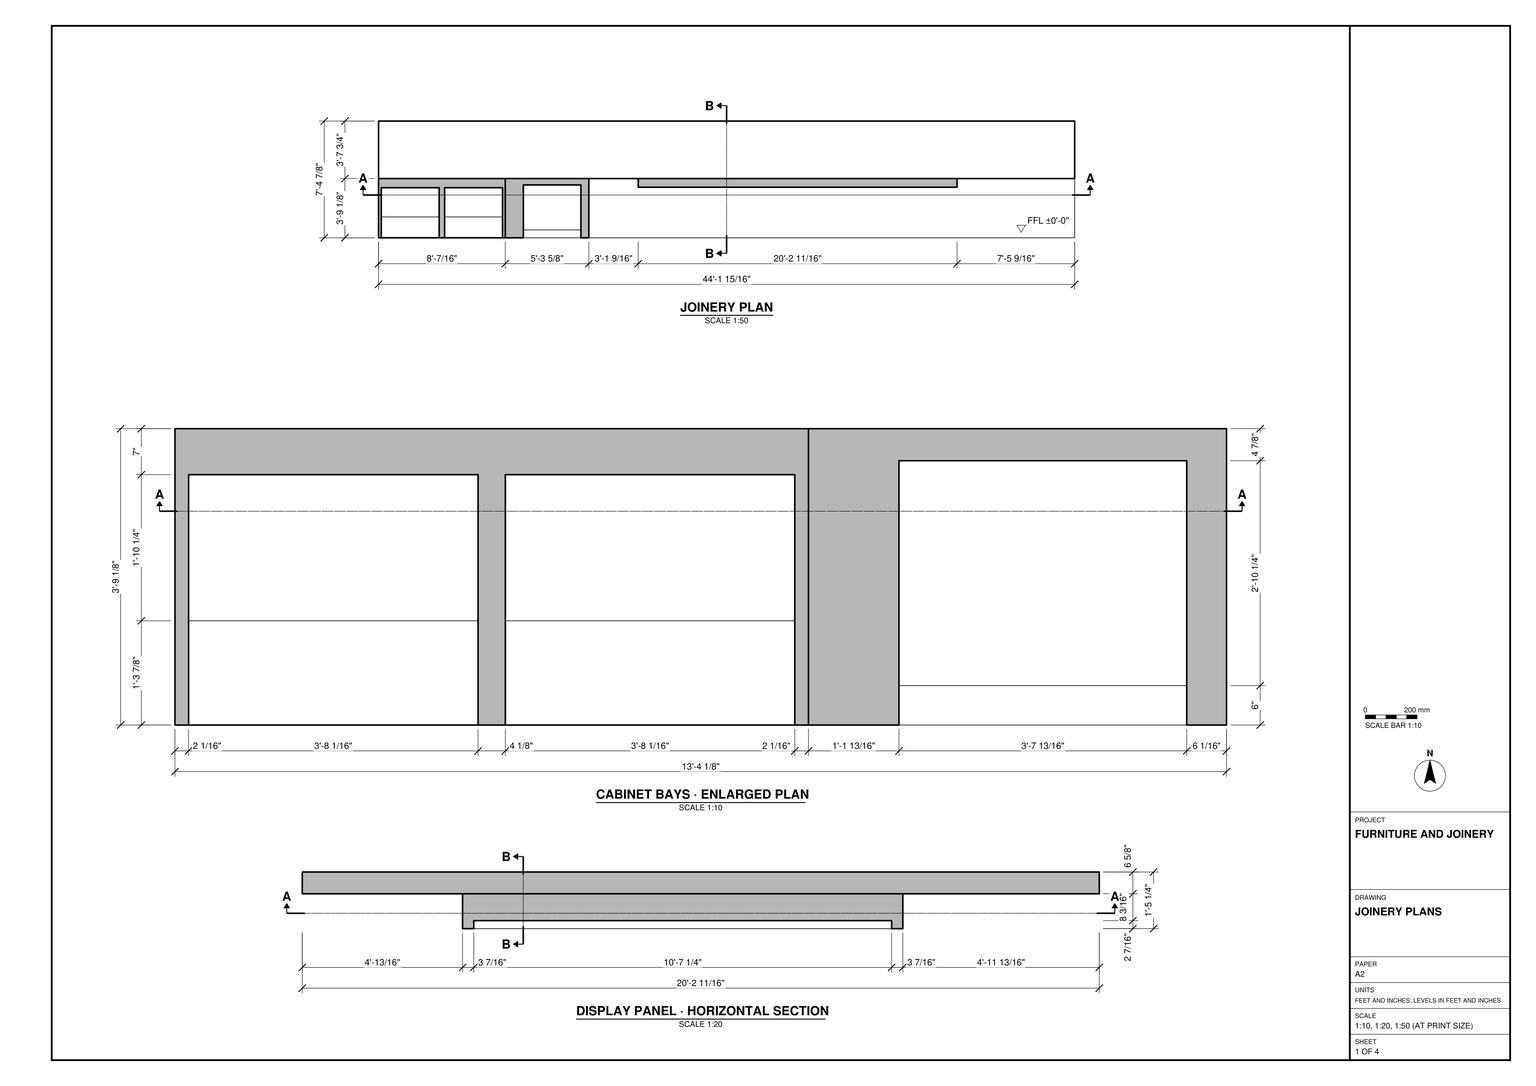
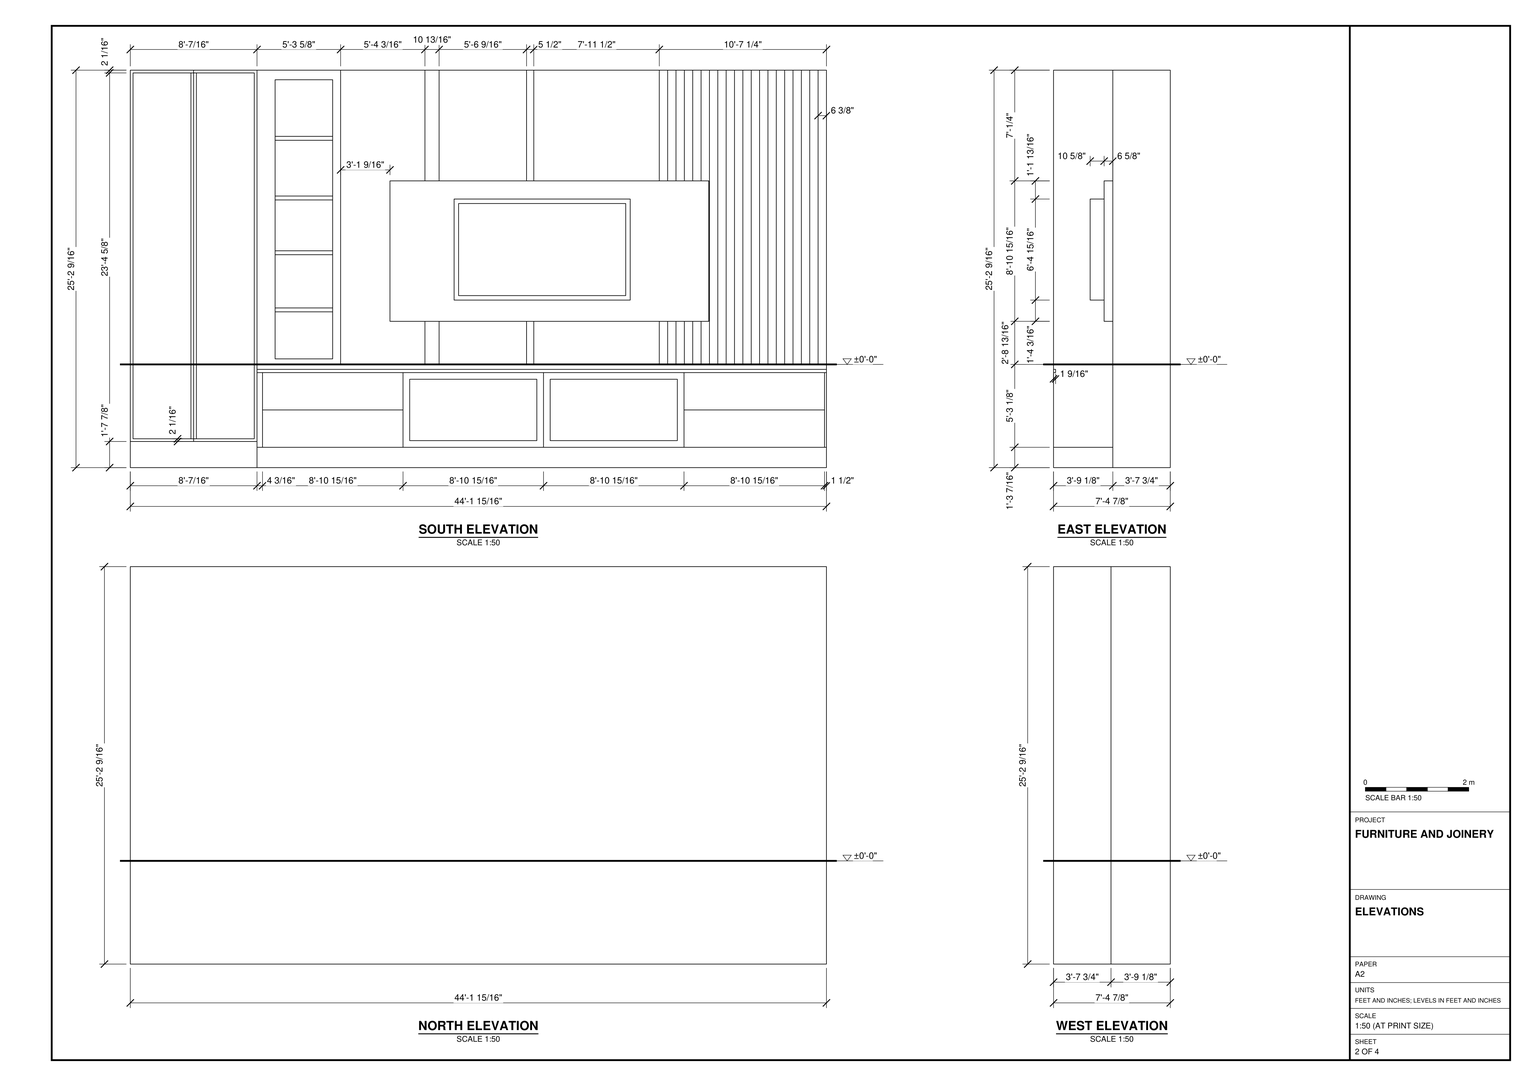
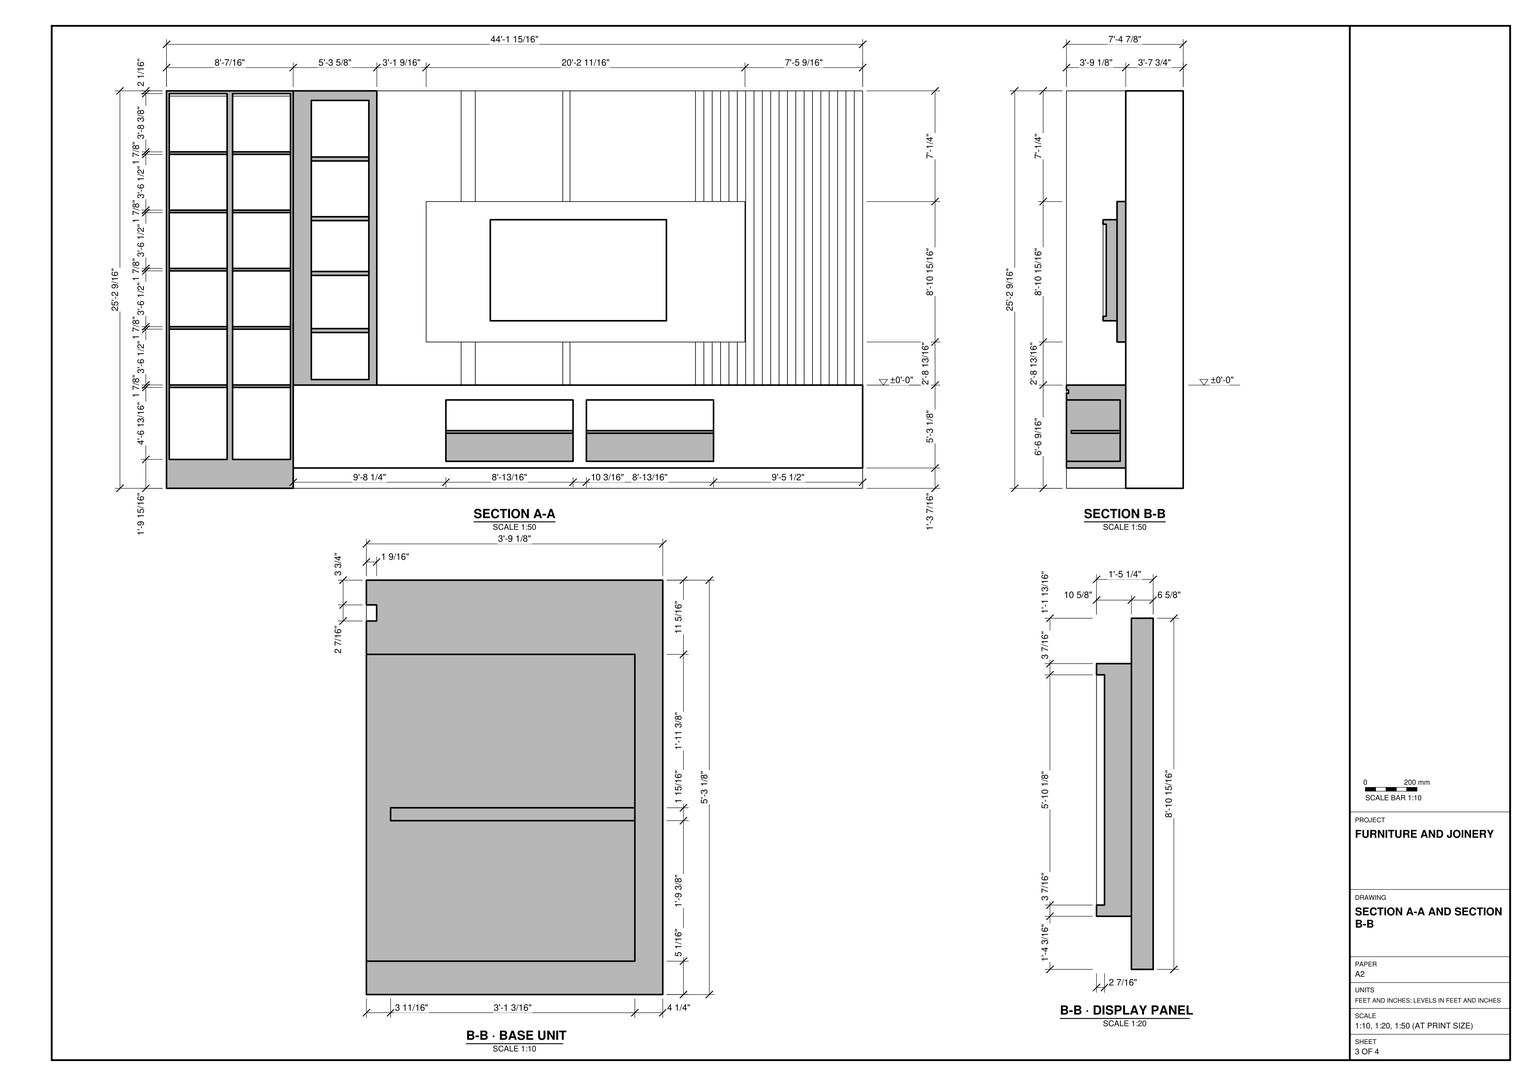
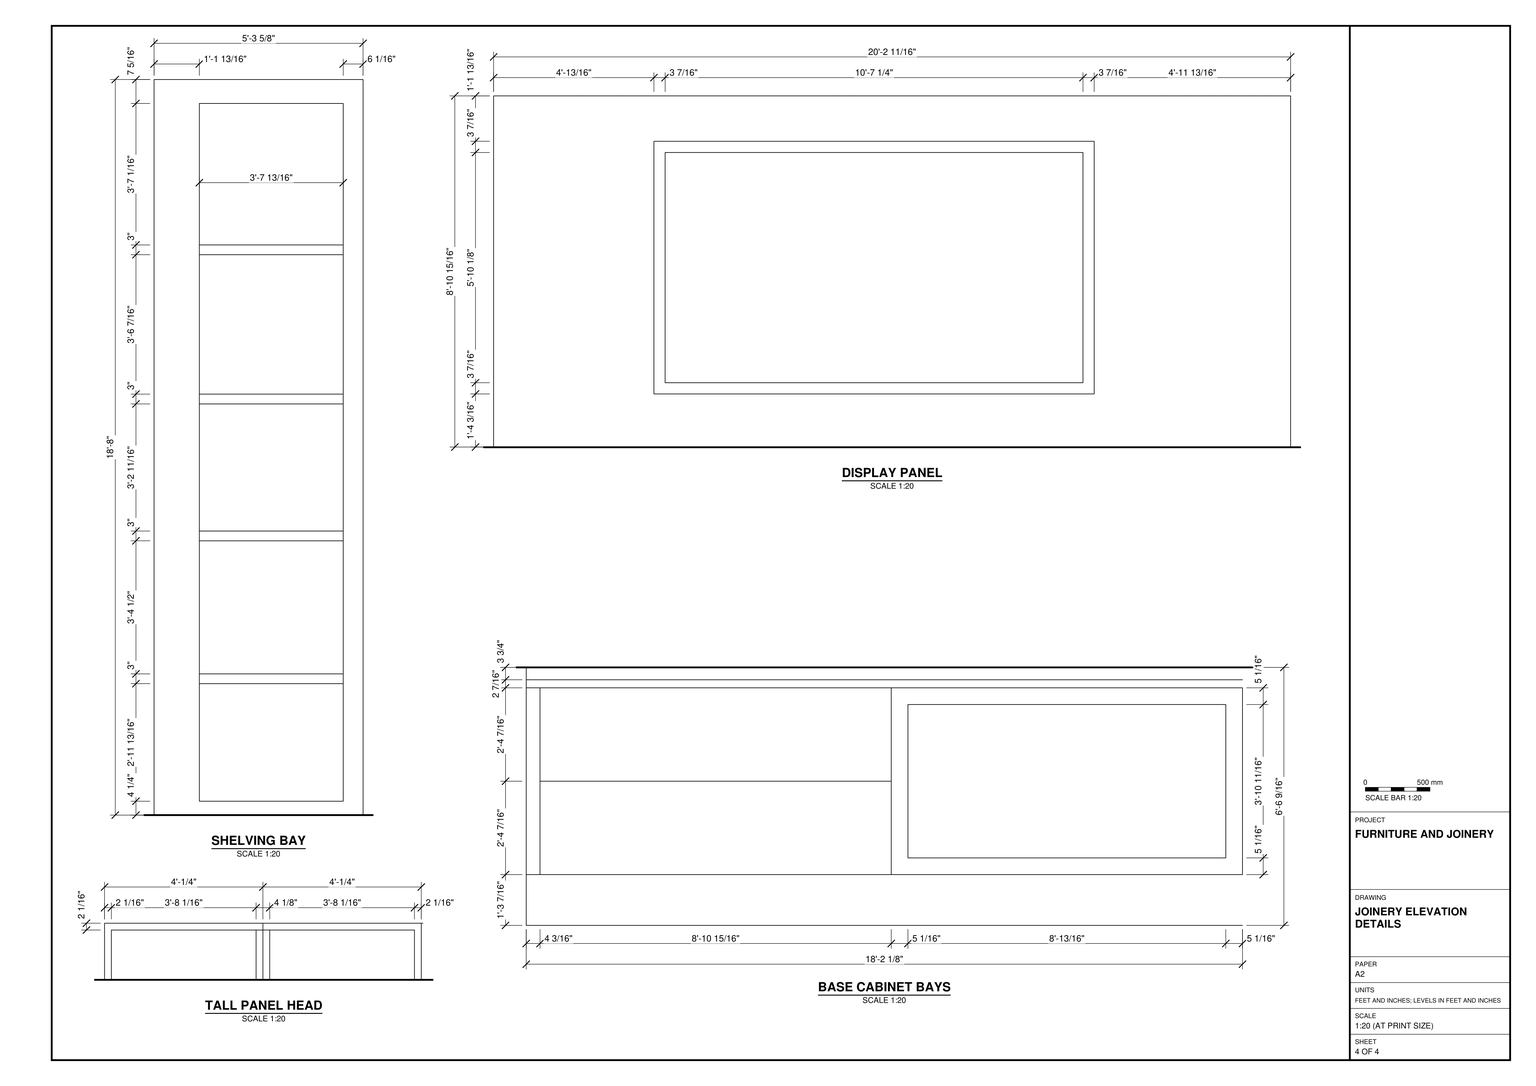
Build the wall joinery in SketchUp from task_files/diagram_01.pdf. Work in feet and inches. The complete assembly is 44'-1 15/16" wide, 7'-4 7/8" deep and 25'-2 9/16" high. Use the single finished-floor datum ±0'-0" as drawn: it aligns with the top of the base cabinet run, not the bottom of the assembly.

Use the south elevation to lay out the front. At the left, model the paired tall cabinet bays and their internal shelves. Place the narrower shelving bay immediately to their right, above the base cabinet. Continue the base cabinet to the right end, matching its front divisions and internal shelf profile to the elevation and sections. Keep the back face plain. On the front of the backing, distinguish the broad vertical panels from the closely spaced vertical strips at the right. Model the wide display panel and its smaller framed face at their respective depths; use the horizontal and vertical sections to set the stepped edges.

Keep the backing, cabinet pieces and display assembly in separate groups or components, and use components for repeated parts. Any decor or loose items shown may use suitable library components. Save one SketchUp model as output_files/display_wall_with_integrated_shelving_and_base_cabinets.skp.

# SketchUp Ruby script. Lengths in inches.
U = 1.inch
M = Sketchup.active_model
def pt(a) = Geom::Point3d.new(a.map { |v| v * U })
def face(e, loops, mat)
  f = e.add_face(loops[0].map { |a| pt(a) })
  loops[1..].each { |l| e.add_face(l.map { |a| pt(a) }).erase! }
  f.material = f.back_material = mat if mat
  f
end
# faces: each face lists its corners as indices into pts; further lists are holes
def faces(e, pts, list, mat = nil) = list.each { |f| face(e, (f[0].is_a?(Array) ? f : [f]).map { |l| l.map { |i| pts[i] } }, mat) }
# xy, xz, yz: faces in a plane at the given z, y or x. An outline is a flat list of corners, or four numbers for a rectangle; further outlines are holes
def ring(l) = l.size == 4 ? [[l[0], l[1]], [l[2], l[1]], [l[2], l[3]], [l[0], l[3]]] : l.each_slice(2).to_a
def flat(e, list, mat, &to3) = list.each { |f| face(e, (f[0].is_a?(Array) ? f : [f]).map { |l| ring(l).map { |u, v| to3.(u, v) } }, mat) }
def xy(e, z, list, mat = nil) = flat(e, list, mat) { |x, y| [x, y, z] }
def xz(e, y, list, mat = nil) = flat(e, list, mat) { |x, z| [x, y, z] }
def yz(e, x, list, mat = nil) = flat(e, list, mat) { |y, z| [x, y, z] }
def lines(e, pts, list) = list.each { |a, b| e.add_line(pt(pts[a]), pt(pts[b])) }
# prism: a flat outline (further loops are holes) pulled along v
def prism(e, loops, v, mat = nil)
  f = face(e, loops, mat); d = Geom::Vector3d.new(v.map { |x| x * U })
  f.pushpull(f.normal.samedirection?(d) ? d.length : -d.length)
end
def box(e, o, s, mat = nil) = prism(e, [[o, [o[0] + s[0], o[1], o[2]], [o[0] + s[0], o[1] + s[1], o[2]], [o[0], o[1] + s[1], o[2]]]], [0, 0, s[2]], mat)
def at(x, y, z, deg = 0) = Geom::Transformation.translation(pt([x, y, z])) * Geom::Transformation.rotation(ORIGIN, Z_AXIS, deg.degrees)
def axes(o, x, y, z) = Geom::Transformation.new([*x, 0, *y, 0, *z, 0, *pt(o).to_a, 1])
def part(name) = M.definitions.add(name)
# library, detail: a bought-in or finely detailed component or shape, given as its bounding box
def library(name, o, s) = part(name).tap { |d| box(d.entities, o, s) }
def detail(e, o, s) = box(e.add_group.entities, o, s)
def put(e, d, t, mat = nil) = e.add_instance(d, t).tap { |i| i.material = mat if mat }
def group(e, t, mat = nil) = e.add_group.tap { |g| g.transformation = t; g.material = mat if mat }.entities
root = M.entities
M.materials.add("[0046_Gold]").color = [255, 215, 0]
M.materials.add("[0081_CadetBlue]").color = [95, 158, 160]
M.materials.add("[0137_Black]").color = [0, 0, 0]
M.materials.add("[Translucent Glass Gray]").color = [128, 128, 128]
M.materials["[Translucent Glass Gray]"].alpha = 0.5
xy(root,39.09,[[0,0,96.45,45.125],[0,45.125,529.9375,88.875]])
xy(root,54.56,[[96.45,0,529.9375,45.125]])
xy(root,59.64,[[212.68,0,309.48,40.875],[319.64,0,416.43,40.875]],"[0081_CadetBlue]")
xy(root,61.06,[[2.08,0,46.15,38.125],[50.3,0,94.37,38.125]],"[0081_CadetBlue]")
xy(root,81.03,[[212.68,3.6875,309.48,40.875],[319.64,3.6875,416.43,40.875]],"[0081_CadetBlue]")
xy(root,82.99,[[212.68,3.6875,309.48,40.875],[319.64,3.6875,416.43,40.875]],"[0081_CadetBlue]")
xy(root,106.35,[[212.68,0,309.48,40.875],[319.64,0,416.43,40.875]])
xy(root,111.43,[[96.45,0,529.9375,1.5625]])
xy(root,113.88,[[96.45,0,529.9375,1.5625]])
xy(root,115.88,[[2.08,15.875,46.15,38.125],[50.3,15.875,94.37,38.125]])
xy(root,117.65,[[96.45,0,160.1,45.125]])
xy(root,117.65,[[160.1,0,529.9375,45.125]],"[0081_CadetBlue]")
xy(root,117.76,[[2.08,15.875,46.15,38.125],[50.3,15.875,94.37,38.125]],"[0081_CadetBlue]")
xy(root,121.875,[[110.23,0,154.05,40.25]],"[0081_CadetBlue]")
xy(root,150.46,[[197.68,38.5,440.36,45.125]])
xy(root,157.68,[[110.23,6,154.05,40.25]],"[0081_CadetBlue]")
xy(root,160.24,[[2.08,15.875,46.15,38.125],[50.3,15.875,94.37,38.125]])
xy(root,160.66,[[110.23,6,154.05,40.25]],"[0081_CadetBlue]")
xy(root,162.125,[[2.08,15.875,46.15,38.125],[50.3,15.875,94.37,38.125]],"[0081_CadetBlue]")
xy(root,166.63,[[246.49,27.875,380.55,38.5]],"[0137_Black]")
xy(root,170.04,[[249.9,27.875,377.14,30.3125]],"[0137_Black]")
xy(root,201.18,[[110.23,6,154.05,40.25]],"[0081_CadetBlue]")
xy(root,204.16,[[110.23,6,154.05,40.25]],"[0081_CadetBlue]")
xy(root,204.61,[[2.08,15.875,46.15,38.125],[50.3,15.875,94.37,38.125]])
xy(root,206.49,[[2.08,15.875,46.15,38.125],[50.3,15.875,94.37,38.125]],"[0081_CadetBlue]")
xy(root,240.16,[[249.9,27.875,377.14,30.3125]])
xy(root,242.87,[[110.23,6,154.05,40.25]],"[0081_CadetBlue]")
xy(root,243.57,[[246.49,27.875,380.55,38.5]],"[0137_Black]")
xy(root,245.85,[[110.23,6,154.05,40.25]],"[0081_CadetBlue]")
xy(root,248.97,[[2.08,15.875,46.15,38.125],[50.3,15.875,94.37,38.125]])
xy(root,250.85,[[2.08,15.875,46.15,38.125],[50.3,15.875,94.37,38.125]],"[0081_CadetBlue]")
xy(root,257.39,[[197.68,38.5,440.36,45.125]])
xy(root,288.3,[[110.23,6,154.05,40.25]],"[0081_CadetBlue]")
xy(root,291.28,[[110.23,6,154.05,40.25]],"[0081_CadetBlue]")
xy(root,293.33,[[2.08,15.875,46.15,38.125],[50.3,15.875,94.37,38.125]])
xy(root,295.21,[[2.08,15.875,46.15,38.125],[50.3,15.875,94.37,38.125]],"[0081_CadetBlue]")
xy(root,334.37,[[110.23,0,154.05,40.25]],"[0081_CadetBlue]")
xy(root,339.57,[[2.08,0,46.15,38.125],[50.3,0,94.37,38.125]],"[0081_CadetBlue]")
xy(root,341.65,[[0,0,96.45,45.125],[96.45,0,160.1,45.125],[0,45.125,529.9375,88.875]],"[0081_CadetBlue]")
xz(root,0,[[96.45,54.56,100.65,111.43],[100.65,54.56,207.6,82.99],[[207.6,54.56,314.56,111.43],[212.68,59.64,309.48,106.35]],[[314.56,54.56,421.51,111.43],[319.64,59.64,416.43,106.35]],[421.51,54.56,528.46,82.99],
  [0,58.98,48.22,58.98,48.22,61.06,2.08,61.06,2.08,339.57,48.22,339.57,48.22,341.65,0,341.65],[48.22,58.98,96.45,58.98,96.45,341.65,48.22,341.65,48.22,339.57,94.37,339.57,94.37,61.06,48.22,61.06],[46.15,61.06,48.22,339.57],[48.22,61.06,50.3,339.57],[100.65,82.99,207.6,111.43],
  [421.51,82.99,528.46,111.43]])
xz(root,0,[[0,39.09,96.45,58.98],[528.46,54.56,529.9375,111.43],[96.45,113.88,529.9375,117.65],[[96.45,117.65,160.1,341.65],[110.23,121.875,154.05,334.37]]],"[0081_CadetBlue]")
xz(root,0,[[212.68,59.64,309.48,106.35],[319.64,59.64,416.43,106.35],[2.08,61.06,46.15,339.57],[50.3,61.06,94.37,339.57]],"[Translucent Glass Gray]")
xz(root,1.5625,[[96.45,111.43,529.9375,113.88]],"[0081_CadetBlue]")
xz(root,3.6875,[[212.68,81.03,309.48,82.99],[319.64,81.03,416.43,82.99]],"[0081_CadetBlue]")
xz(root,6,[[110.23,157.68,154.05,160.66],[110.23,201.18,154.05,204.16],[110.23,242.87,154.05,245.85],[110.23,288.3,154.05,291.28]],"[0081_CadetBlue]")
xz(root,15.875,[[2.08,115.88,46.15,117.76],[50.3,115.88,94.37,117.76],[2.08,160.24,46.15,162.125],[50.3,160.24,94.37,162.125],[2.08,204.61,46.15,206.49],
  [50.3,204.61,94.37,206.49],[2.08,248.97,46.15,250.85],[50.3,248.97,94.37,250.85],[2.08,293.33,46.15,295.21],[50.3,293.33,94.37,295.21]])
xz(root,27.875,[[[246.49,166.63,380.55,243.57],[249.9,170.04,377.14,240.16]]],"[0137_Black]")
xz(root,30.3125,[[249.9,170.04,377.14,240.16]],"[0137_Black]")
xz(root,38.125,[[2.08,61.06,46.15,115.88],[50.3,61.06,94.37,115.88],[2.08,115.88,46.15,117.76],[50.3,115.88,94.37,117.76],[2.08,117.76,46.15,160.24],
  [50.3,117.76,94.37,160.24],[2.08,160.24,46.15,162.125],[50.3,160.24,94.37,162.125],[2.08,162.125,46.15,204.61],[50.3,162.125,94.37,204.61],
  [2.08,204.61,46.15,206.49],[50.3,204.61,94.37,206.49],[2.08,206.49,46.15,248.97],[50.3,206.49,94.37,248.97],[2.08,248.97,46.15,250.85],
  [50.3,248.97,94.37,250.85],[2.08,250.85,46.15,293.33],[50.3,250.85,94.37,293.33],[2.08,293.33,46.15,295.21],[50.3,293.33,94.37,295.21],
  [2.08,295.21,46.15,337.69],[50.3,295.21,94.37,337.69],[2.08,337.69,46.15,339.57],[50.3,337.69,94.37,339.57]])
xz(root,38.5,[[[197.68,150.46,440.36,257.39],[246.49,166.63,380.55,243.57]],[246.49,166.63,380.55,243.57]])
xz(root,40.25,[[110.23,157.68,154.05,160.66],[110.23,201.18,154.05,204.16],[110.23,242.87,154.05,245.85],[110.23,288.3,154.05,291.28]])
xz(root,40.25,[[110.23,121.875,154.05,157.68],[110.23,160.66,154.05,201.18],[110.23,204.16,154.05,242.87],[110.23,245.85,154.05,288.3],[110.23,291.28,154.05,334.37]],"[0081_CadetBlue]")
xz(root,40.875,[[212.68,81.03,309.48,82.99],[319.64,81.03,416.43,82.99]])
xz(root,40.875,[[212.68,59.64,309.48,81.03],[319.64,59.64,416.43,81.03],[212.68,82.99,309.48,106.35],[319.64,82.99,416.43,106.35]],"[0081_CadetBlue]")
xz(root,45.125,[[0,39.09,96.45,341.65],[96.45,39.09,529.9375,54.56],[96.45,54.56,529.9375,117.65],[96.45,117.65,160.1,341.65],[160.1,117.65,224.28,117.65,224.28,150.46,197.68,150.46,197.68,257.39,224.28,257.39,224.28,341.65,160.1,341.65],
  [235.07,117.65,301.66,150.46],[307.16,117.65,402.6875,150.46],[402.6875,117.65,409.05,150.46],[197.68,150.46,402.6875,257.39],[402.6875,150.46,409.05,257.39],
  [409.05,150.46,415.41,257.39],[415.41,150.46,421.77,257.39],[421.77,150.46,428.14,257.39],[428.14,150.46,434.5,257.39],[434.5,150.46,440.36,257.39],
  [235.07,257.39,301.66,341.65],[307.16,257.39,402.6875,341.65]])
xz(root,45.125,[[224.28,117.65,235.07,150.46],[301.66,117.65,307.16,150.46],[224.28,257.39,235.07,341.65],[301.66,257.39,307.16,341.65]],"[0046_Gold]")
xz(root,45.125,[[409.05,117.65,415.41,150.46],[415.41,117.65,421.77,150.46],[421.77,117.65,428.14,150.46],[428.14,117.65,434.5,150.46],[434.5,117.65,440.86,117.65,440.86,341.65,434.5,341.65,434.5,257.39,440.36,257.39,440.36,150.46,434.5,150.46],
  [440.86,117.65,447.23,341.65],[447.23,117.65,453.59,341.65],[453.59,117.65,459.95,341.65],[459.95,117.65,466.3125,341.65],[466.3125,117.65,472.67,341.65],
  [472.67,117.65,479.04,341.65],[479.04,117.65,485.4,341.65],[485.4,117.65,491.76,341.65],[491.76,117.65,498.125,341.65],[498.125,117.65,504.49,341.65],
  [504.49,117.65,510.85,341.65],[510.85,117.65,517.21,341.65],[517.21,117.65,523.58,341.65],[523.58,117.65,529.9375,341.65],[402.6875,257.39,409.05,341.65],
  [409.05,257.39,415.41,341.65],[415.41,257.39,421.77,341.65],[421.77,257.39,428.14,341.65],[428.14,257.39,434.5,341.65]],"[0081_CadetBlue]")
xz(root,88.875,[[0,39.09,529.9375,341.65]])
yz(root,0,[[0,39.09,45.125,341.65],[45.125,39.09,88.875,341.65]])
yz(root,2.08,[[0,61.06,38.125,61.06,38.125,115.88,15.875,115.88,15.875,117.76,38.125,117.76,38.125,160.24,15.875,160.24,15.875,162.125,38.125,162.125,38.125,204.61,15.875,204.61,15.875,206.49,38.125,206.49,38.125,248.97,15.875,248.97,15.875,250.85,38.125,250.85,38.125,293.33,15.875,293.33,15.875,295.21,38.125,295.21,38.125,339.57,0,339.57],[15.875,115.88,38.125,117.76],[15.875,160.24,38.125,162.125],[15.875,204.61,38.125,206.49],[15.875,248.97,38.125,250.85],
  [15.875,293.33,38.125,295.21]])
yz(root,46.15,[[0,61.06,0,339.57,38.125,339.57,38.125,295.21,15.875,295.21,15.875,293.33,38.125,293.33,38.125,250.85,15.875,250.85,15.875,248.97,38.125,248.97,38.125,206.49,15.875,206.49,15.875,204.61,38.125,204.61,38.125,162.125,15.875,162.125,15.875,160.24,38.125,160.24,38.125,117.76,15.875,117.76,15.875,115.88,38.125,115.88,38.125,61.06],[15.875,115.88,38.125,117.76],[15.875,160.24,38.125,162.125],[15.875,204.61,38.125,206.49],[15.875,248.97,38.125,250.85],
  [15.875,293.33,38.125,295.21]])
yz(root,50.3,[[0,61.06,38.125,61.06,38.125,115.88,15.875,115.88,15.875,117.76,38.125,117.76,38.125,160.24,15.875,160.24,15.875,162.125,38.125,162.125,38.125,204.61,15.875,204.61,15.875,206.49,38.125,206.49,38.125,248.97,15.875,248.97,15.875,250.85,38.125,250.85,38.125,293.33,15.875,293.33,15.875,295.21,38.125,295.21,38.125,339.57,0,339.57],[15.875,115.88,38.125,117.76],[15.875,160.24,38.125,162.125],[15.875,204.61,38.125,206.49],[15.875,248.97,38.125,250.85],
  [15.875,293.33,38.125,295.21]])
yz(root,94.37,[[0,61.06,0,117.65,15.875,117.65,15.875,115.88,38.125,115.88,38.125,61.06],[15.875,115.88,38.125,117.65],[0,117.65,0,339.57,38.125,339.57,38.125,295.21,15.875,295.21,15.875,293.33,38.125,293.33,38.125,250.85,15.875,250.85,15.875,248.97,38.125,248.97,38.125,206.49,15.875,206.49,15.875,204.61,38.125,204.61,38.125,162.125,15.875,162.125,15.875,160.24,38.125,160.24,38.125,117.76,15.875,117.76,15.875,117.65],[15.875,117.65,38.125,117.76],[15.875,160.24,38.125,162.125],
  [15.875,204.61,38.125,206.49],[15.875,248.97,38.125,250.85],[15.875,293.33,38.125,295.21]])
yz(root,96.45,[[0,39.09,45.125,54.56],[0,54.56,45.125,54.56,45.125,117.65,0,117.65,0,113.88,1.5625,113.88,1.5625,111.43,0,111.43],[0,111.43,1.5625,113.88],[0,117.65,45.125,341.65]])
yz(root,110.23,[[6,157.68,40.25,160.66],[6,201.18,40.25,204.16],[6,242.87,40.25,245.85],[6,288.3,40.25,291.28]])
yz(root,110.23,[[0,121.875,40.25,121.875,40.25,157.68,6,157.68,6,160.66,40.25,160.66,40.25,201.18,6,201.18,6,204.16,40.25,204.16,40.25,242.87,6,242.87,6,245.85,40.25,245.85,40.25,288.3,6,288.3,6,291.28,40.25,291.28,40.25,334.37,0,334.37]],"[0081_CadetBlue]")
yz(root,154.05,[[6,157.68,40.25,160.66],[6,201.18,40.25,204.16],[6,242.87,40.25,245.85],[6,288.3,40.25,291.28]])
yz(root,154.05,[[0,121.875,0,334.37,40.25,334.37,40.25,291.28,6,291.28,6,288.3,40.25,288.3,40.25,245.85,6,245.85,6,242.87,40.25,242.87,40.25,204.16,6,204.16,6,201.18,40.25,201.18,40.25,160.66,6,160.66,6,157.68,40.25,157.68,40.25,121.875]],"[0081_CadetBlue]")
yz(root,160.1,[[0,117.65,45.125,341.65]],"[0081_CadetBlue]")
yz(root,197.68,[[38.5,150.46,45.125,257.39]])
yz(root,212.68,[[3.6875,81.03,40.875,82.99]])
yz(root,212.68,[[0,59.64,40.875,59.64,40.875,81.03,3.6875,81.03,3.6875,82.99,40.875,82.99,40.875,106.35,0,106.35]],"[0081_CadetBlue]")
yz(root,246.49,[[27.875,166.63,38.5,243.57]],"[0137_Black]")
yz(root,249.9,[[27.875,170.04,30.3125,240.16]],"[0137_Black]")
yz(root,309.48,[[3.6875,81.03,40.875,82.99]])
yz(root,309.48,[[0,59.64,0,106.35,40.875,106.35,40.875,82.99,3.6875,82.99,3.6875,81.03,40.875,81.03,40.875,59.64]],"[0081_CadetBlue]")
yz(root,319.64,[[0,59.64,40.875,59.64,40.875,81.03,3.6875,81.03,3.6875,82.99,40.875,82.99,40.875,106.35,0,106.35],[3.6875,81.03,40.875,82.99]])
yz(root,377.14,[[27.875,170.04,30.3125,240.16]],"[0137_Black]")
yz(root,380.55,[[27.875,166.63,38.5,243.57]],"[0137_Black]")
yz(root,416.43,[[3.6875,81.03,40.875,82.99]])
yz(root,416.43,[[0,59.64,0,106.35,40.875,106.35,40.875,82.99,3.6875,82.99,3.6875,81.03,40.875,81.03,40.875,59.64]],"[0081_CadetBlue]")
yz(root,440.36,[[38.5,150.46,45.125,257.39]])
yz(root,529.9375,[[45.125,39.09,88.875,341.65]])
yz(root,529.9375,[[0,54.56,45.125,54.56,45.125,117.65,0,117.65,0,113.88,1.5625,113.88,1.5625,111.43,0,111.43]],"[0081_CadetBlue]")
